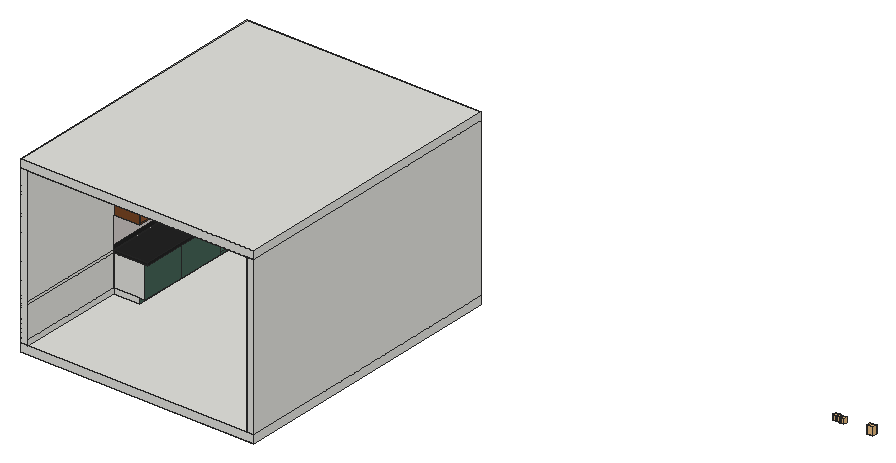
# SketchUp Ruby script. Lengths in inches.
U = 1.inch
M = Sketchup.active_model
def pt(a) = Geom::Point3d.new(a.map { |v| v * U })
def face(e, loops, mat)
  f = e.add_face(loops[0].map { |a| pt(a) })
  loops[1..].each { |l| e.add_face(l.map { |a| pt(a) }).erase! }
  f.material = f.back_material = mat if mat
  f
end
# faces: each face lists its corners as indices into pts; further lists are holes
def faces(e, pts, list, mat = nil) = list.each { |f| face(e, (f[0].is_a?(Array) ? f : [f]).map { |l| l.map { |i| pts[i] } }, mat) }
# xy, xz, yz: faces in a plane at the given z, y or x. An outline is a flat list of corners, or four numbers for a rectangle; further outlines are holes
def ring(l) = l.size == 4 ? [[l[0], l[1]], [l[2], l[1]], [l[2], l[3]], [l[0], l[3]]] : l.each_slice(2).to_a
def flat(e, list, mat, &to3) = list.each { |f| face(e, (f[0].is_a?(Array) ? f : [f]).map { |l| ring(l).map { |u, v| to3.(u, v) } }, mat) }
def xy(e, z, list, mat = nil) = flat(e, list, mat) { |x, y| [x, y, z] }
def xz(e, y, list, mat = nil) = flat(e, list, mat) { |x, z| [x, y, z] }
def yz(e, x, list, mat = nil) = flat(e, list, mat) { |y, z| [x, y, z] }
def lines(e, pts, list) = list.each { |a, b| e.add_line(pt(pts[a]), pt(pts[b])) }
# prism: a flat outline (further loops are holes) pulled along v
def prism(e, loops, v, mat = nil)
  f = face(e, loops, mat); d = Geom::Vector3d.new(v.map { |x| x * U })
  f.pushpull(f.normal.samedirection?(d) ? d.length : -d.length)
end
def box(e, o, s, mat = nil) = prism(e, [[o, [o[0] + s[0], o[1], o[2]], [o[0] + s[0], o[1] + s[1], o[2]], [o[0], o[1] + s[1], o[2]]]], [0, 0, s[2]], mat)
def at(x, y, z, deg = 0) = Geom::Transformation.translation(pt([x, y, z])) * Geom::Transformation.rotation(ORIGIN, Z_AXIS, deg.degrees)
def axes(o, x, y, z) = Geom::Transformation.new([*x, 0, *y, 0, *z, 0, *pt(o).to_a, 1])
def part(name) = M.definitions.add(name)
# library, detail: a bought-in or finely detailed component or shape, given as its bounding box
def library(name, o, s) = part(name).tap { |d| box(d.entities, o, s) }
def detail(e, o, s) = box(e.add_group.entities, o, s)
def put(e, d, t, mat = nil) = e.add_instance(d, t).tap { |i| i.material = mat if mat }
def group(e, t, mat = nil) = e.add_group.tap { |g| g.transformation = t; g.material = mat if mat }.entities
root = M.entities
M.materials.add("4 (5)").color = [147, 109, 57]
M.materials.add("[0012_Bisque]").color = [255, 228, 196]
M.materials.add("[0136_Charcoal]").color = [35, 35, 35]
M.materials.add("[0137_Black]").color = [0, 0, 0]
M.materials.add("[Color C07]").color = [153, 76, 0]
M.materials["[Color C07]"].alpha = 0.27
M.materials.add("[Color G02]").color = [68, 99, 86]
M.materials.add("[Color M08]").color = [30, 30, 30]
M.materials.add("[Tile Hexagon White]").color = [213, 206, 204]
M.materials.add("[Wood Veneer 01]").color = [120, 70, 37]
c1 = part("Group\#46")
prism(c1.entities,[[[0.55,0,1.11],[0.51,0,1.03],[0.44,0,0.97],[0.36,0,0.9375],[0.28,0,0.92],[0.19,0,0.9375],[0.11,0,0.97],[0.05,0,1.03],[0,0,1.11],[0,0,0],[0.55,0,0]]],[0,0.79,0])
c2 = part("Cabinet pull handle")
put(c2.entities,c1,axes([0,1.42,1.36],[0,0,-1],[1,0,0],[0,-1,0]))
g1 = group(c2.entities,at(0,1.42,1.36))
prism(g1,[[[0,-1.28,-0.57],[0,-1.32,-0.53],[0,-1.35,-0.49],[0,-1.38,-0.4375],[0,-1.4,-0.39],[0,-1.41,-0.33],[0,-1.42,-0.28],[0,-1.41,-0.22],[0,-1.4,-0.17],[0,-1.38,-0.11],[0,-1.35,-0.0625],[0,-1.32,-0.02],[0,-1.28,0.02],[0,-1.19,0.02],[0,-1.11,0],[0,-1.03,-0.05],[0,-0.97,-0.11],[0,-0.9375,-0.19],[0,-0.92,-0.28],[0,-0.9375,-0.36],[0,-0.97,-0.44],[0,-1.03,-0.51],[0,-1.11,-0.55],[0,-1.19,-0.57]]],[13.07,0,0])
put(c2.entities,c1,axes([12.28,1.42,1.36],[0,0,-1],[1,0,0],[0,-1,0]))
c3 = library("Food+jars (1)",[-3.15,-4.1,0],[15.4,16.05,11.47])
c4 = library("Stack of bowls \#1",[0,0,0],[8.98,8.99,10.96])
c5 = library("jars",[-134.79,-4.32,0],[83.43,13.28,34.83])
c6 = library("KITCHEN+ITEMS+(3)",[-2.27,-9.02,0],[4.03,10.9,5.45])
c7 = library("filizanka,+spodek+zestaw",[-38.08,-53.17,0],[37.3,56.83,6.3])
c8 = library("Food+jars",[176.18,154.2,55.15],[6.14,23.65,7.76])
c9 = library("Component_12",[0,0,0],[17.72,31.5,20.63])
c10 = library("1045",[78.33,40.52,-0.08],[23.62,20.2,1.2])
c11 = library("PV977NSS_GEProfile",[-17.9375,-27.5625,-0.25],[35.95,27.64,32.08])
c12 = part("Sink basin")
detail(c12.entities,[-0.15,-0.15,0],[19.98,14.07,5.91])
c13 = part("Untitled (26)")
put(c13.entities,c12,at(0.15,0.15,0),"4 (5)")
c14 = library("Group\#21",[-462.66,84.21,613.65],[72.44,72.44,111.8])
c15 = library("Group\#23",[-457.8,68.7,378.69],[103.44,103.46,159.72])
c16 = library("Group\#22",[-210.76,89.58,378.69],[103.46,103.45,159.72])
c17 = library("Group\#24",[-332.7,68.71,378.69],[103.45,103.45,159.72])
c18 = library("Group\#15",[-374.05,84.21,613.65],[72.44,72.44,111.8])
c19 = library("Group\#14",[-289.4,84.22,613.65],[72.44,72.43,111.8])
c20 = library("Group\#13",[-92.73,64.66,378.72],[126.77,111.9,197.69])
c21 = library("Group\#9",[51.24,128.79,378.72],[113.79,95.47,197.69])
c22 = library("Group\#10",[179.9,72.7,378.72],[113.8,95.46,197.69])
c23 = library("Group\#11",[327.72,72.7,378.72],[113.79,95.46,197.69])
c24 = library("Group\#12",[309.63,77.04,613.73],[136.79,86.78,171.39])
c25 = library("Group\#25",[0,0,0],[16.24,2.86,5.88])
xy(root,-6,[[0,0,178.59,216.47]])
xy(root,0,[[0,0,5.86,0,5.86,81.5625,25.86,81.5625,25.86,190.14,5.92,190.07,5.86,210.07,5.86,210.61,172.73,210.61,172.8,190.61,172.73,190.61,172.73,0,178.59,0,178.59,216.47,0,216.47],[5.86,0,172.73,0,172.73,190.61,29.92,190.15,25.86,190.14,25.86,81.5625,5.86,81.5625],[5.92,190.07,25.86,190.14,25.86,210.07,5.86,210.07],[25.86,190.14,25.86,210.07,29.86,210.07,29.92,190.15],[29.92,190.15,172.73,190.61,172.73,210.07,29.86,210.07],
  [172.73,190.61,172.73,210.61,172.8,190.61],[5.86,210.07,29.86,210.15,29.86,210.07],[5.86,210.07,5.86,210.61,29.86,210.61,29.86,210.15],[29.86,210.07,172.73,210.15],[29.86,210.15,172.73,210.15,172.73,210.61],
  [29.86,210.15,29.86,210.61,172.73,210.61]])
xy(root,0.4375,[[29.86,190.15,172.73,190.61,172.73,190.15],[29.86,190.15,172.73,190.61,172.73,210.07,29.86,210.07],[172.73,190.61,172.8,190.61,172.73,210.61,5.86,210.07,172.73,210.07]])
xy(root,4,[[5.86,81.5625,5.86,210.07,5.92,190.07,25.86,190.14,25.86,81.5625],[25.86,81.5625,25.86,190.14,29.86,190.15,29.86,81.5625],[29.86,188.15,172.73,190.15],[5.92,190.07,25.86,190.14,25.86,210.07,5.86,210.07],[25.86,190.14,25.86,210.07,29.86,210.07,29.86,190.15],
  [29.86,190.15,172.73,210.07]])
xy(root,4.67,[[9.42,153.29,29.86,187.48]],"[Color G02]")
xy(root,12.39,[[31.11,188.15,65.58,188.46],[65.58,188.15,101.3,188.46]])
xy(root,12.6875,[[31.11,188.15,65.58,188.46],[65.58,188.15,101.3,188.46]])
xy(root,16,[[9.42,153.29,29.86,187.48]])
xy(root,16.67,[[9.42,153.29,29.86,187.48]],"[Color G02]")
xy(root,20.25,[[31.86,190.15,172.73,210.61]])
xy(root,20.77,[[31.11,188.15,65.58,188.53],[65.58,188.15,101.3,188.46]])
xy(root,21.07,[[31.11,188.15,65.58,188.53],[65.58,188.15,101.3,188.46]])
xy(root,23,[[136.1,188.6,163.66,208.78]])
xy(root,27.33,[[9.42,153.29,29.86,187.48]])
xy(root,28,[[5.86,81.5625,29.86,210.61],[29.86,81.5625,31.86,188.15],[31.86,184.61,172.73,188.15],[29.86,188.15,31.86,190.15],[31.86,188.15,172.73,190.15],
  [29.86,190.15,31.86,210.61]])
xy(root,30,[[[5.86,81.5625,31.86,81.5625,31.86,184.61,172.73,184.61,172.73,210.61,5.86,210.61],[136.1,188.6,163.66,208.78]]],"[0136_Charcoal]")
xy(root,54,[[5.86,81.5625,25.86,210.61],[98.11,197.13,172.73,210.61],[25.86,197.48,60.23,210.61]],"[Wood Veneer 01]")
xy(root,54.4,[[98.11,197.13,98.51,197.14]])
xy(root,54.4,[[98.51,197.13,172.73,197.13,172.73,197.44,172.33,197.44,172.33,212.98,98.51,212.98]],"[Wood Veneer 01]")
xy(root,54.6,[[1.8,82.18,25.86,82.18,25.86,197.14,59.63,197.14,59.63,212.98,1.8,212.98]],"[Wood Veneer 01]")
xy(root,65.38,[[1.8,82.18,25.86,108.82],[1.8,108.82,25.86,136.09],[1.8,136.09,25.86,163.35],[1.8,163.35,25.86,190.61]],"[Wood Veneer 01]")
xy(root,65.4,[[1.8,190.61,59.63,212.98]],"[Wood Veneer 01]")
xy(root,65.6,[[98.51,190.61,117.8,212.98],[117.8,190.61,136.3,212.98],[136.3,190.61,155.11,212.98],[155.11,190.61,172.33,212.98]],"[Wood Veneer 01]")
xy(root,66,[[60.23,190.61,98.11,210.61]])
xy(root,66.67,[[1.8,109.5,25.86,162.67]])
xy(root,66.82,[[98.92,190.61,135.48,212.98]])
xy(root,67.18,[[27.03,190.61,59.06,212.98]])
xy(root,76.6,[[1.8,109.5,25.3,162.67]])
xy(root,77.39,[[98.92,193.17,135.48,212.98]])
xy(root,78,[[1.8,109.5,25.3,162.67],[98.92,193.17,135.48,212.98]])
xy(root,78.8125,[[27.03,192.23,59.06,212.98]])
xy(root,79.375,[[27.03,192.23,59.06,212.98]])
xy(root,88.82,[[27.03,190.61,59.06,212.98]])
xy(root,89.18,[[98.92,190.61,135.48,212.98]])
xy(root,89.33,[[1.8,109.5,25.86,162.67]])
xy(root,90,[[25.86,81.5625,33.3,186.61],[33.3,183.17,33.3,186.61,25.86,186.61,25.86,190.61,172.73,190.61,172.73,183.17]],"[Wood Veneer 01]")
xy(root,92,[[29.86,81.5625,33.3,186.61],[33.3,183.17,172.73,186.61]])
xy(root,120,[[0,0,0,216.47,178.59,216.47,178.59,0,172.73,0,172.73,186.61,29.86,186.61,29.86,81.5625,5.86,81.5625,5.86,0],[5.86,0,5.86,81.5625,29.86,81.5625,29.86,186.61,172.73,186.61,172.73,0]])
xy(root,126,[[0,0,178.59,216.47]])
xz(root,0,[[0,-6,178.59,0],[0,0,5.86,120],[172.73,0,178.59,120],[0,120,178.59,126]])
xz(root,81.5625,[[5.86,0,25.86,4],[5.86,4,29.86,28],[25.86,66,25.86,90,5.86,90,5.86,66.67],[5.86,90,33.3,92],[5.86,92,29.86,120]])
xz(root,81.5625,[[5.86,28,31.86,30]],"[0136_Charcoal]")
xz(root,81.5625,[[5.86,54,25.86,54,25.86,66,5.86,66.67]],"[Wood Veneer 01]")
xz(root,82.18,[[1.8,54.6,25.86,65.38]])
xz(root,109.5,[[1.8,66.67,25.86,76.6],[25.3,76.6,25.86,78],[1.8,78,25.86,89.33]])
xz(root,153.29,[[9.42,4.67,29.86,16],[9.42,16,29.86,16.67],[9.42,16.67,29.86,27.33]])
xz(root,162.67,[[1.8,66.67,25.86,76.6],[25.3,76.6,25.86,78],[1.8,78,25.86,89.33]])
xz(root,183.17,[[33.3,90,172.73,92]],"[Wood Veneer 01]")
xz(root,184.61,[[31.86,28,172.73,30]],"[0137_Black]")
xz(root,186.61,[[33.3,92,33.6,120],[77.48,92,77.78,120],[125.11,92,125.41,120]])
xz(root,186.61,[[29.86,92,33.3,120],[33.6,92,77.48,120],[77.78,92,125.11,120],[125.41,92,172.73,120]],"[0012_Bisque]")
xz(root,187.48,[[9.42,4.67,29.86,16],[9.42,16.67,29.86,27.33]],"[Color G02]")
xz(root,188.15,[[29.86,4,31.11,28],[31.11,4,65.58,12.39],[65.58,4,101.3,12.39],[101.3,4,137.01,28],[137.01,4,172.73,28],
  [31.11,12.6875,65.58,20.77],[65.58,12.6875,101.3,20.77],[31.11,21.07,65.58,28],[65.58,21.07,101.3,28]],"[Color G02]")
xz(root,188.46,[[31.11,12.39,65.58,12.6875],[65.58,12.39,101.3,12.6875],[65.58,20.77,101.3,21.07]])
xz(root,188.53,[[31.11,20.77,65.58,21.07]])
xz(root,188.6,[[136.1,23,163.66,30]])
xz(root,190.15,[[29.86,4,29.86,28,31.86,28,31.86,20.25,172.73,20.25,172.73,4],[31.86,20.25,172.73,28]])
xz(root,190.15,[[29.86,0.4375,172.73,4]],"[Color G02]")
xz(root,190.61,[[1.8,65.38,25.86,65.4],[25.86,65.4,59.63,66],[155.11,66,155.41,90]])
xz(root,190.61,[[60.23,66,98.11,90]],"[0012_Bisque]")
xz(root,190.61,[[136.3,66,155.11,90],[155.41,66,172.73,90]],"[Color G02]")
xz(root,190.61,[[[25.86,66,60.23,90],[27.03,67.18,59.06,88.82]],[[98.11,66,136.3,90],[98.92,66.82,135.48,89.18]]],"[Color M08]")
xz(root,190.61,[[98.51,65.6,172.73,66]],"[Wood Veneer 01]")
xz(root,192.23,[[27.03,78.8125,59.06,79.375]])
xz(root,193.17,[[98.92,77.39,135.48,78]])
xz(root,197.13,[[98.11,54,172.73,54.4]],"[Wood Veneer 01]")
xz(root,197.14,[[98.11,54.4,98.51,54.6]])
xz(root,208.78,[[136.1,23,163.66,30]])
xz(root,210.07,[[5.86,0,25.86,0.4375],[25.86,0,29.86,0.4375],[29.86,0,172.73,0.4375],[5.86,0.4375,25.86,4],[25.86,0.4375,29.86,4],
  [29.86,0.4375,172.73,4]])
xz(root,210.61,[[5.86,0,29.86,28],[29.86,0,172.73,0,172.73,20.25,31.86,20.25,31.86,28,29.86,28],[31.86,20.25,172.73,30],[5.86,28,31.86,30]])
xz(root,210.61,[[5.86,30,172.73,33.57]],"[0136_Charcoal]")
xz(root,210.61,[[5.86,33.57,172.73,33.57,172.73,54,98.11,54,98.11,66,60.23,66,60.23,54,5.86,54]],"[Tile Hexagon White]")
xz(root,212.98,[[98.92,66.82,135.48,77.39],[27.03,67.18,59.06,78.8125],[98.92,78,135.48,89.18],[27.03,79.375,59.06,88.82]])
xz(root,212.98,[[98.51,54.4,172.33,65.6],[1.8,54.6,59.63,65.4]],"[Wood Veneer 01]")
xz(root,216.47,[[0,-6,178.59,0],[0,0,178.59,120],[0,120,178.59,126]])
yz(root,0,[[0,-6,216.47,0],[0,0,216.47,120],[0,120,216.47,126]])
yz(root,1.8,[[109.5,66.67,162.67,76.6],[109.5,78,162.67,89.33]])
yz(root,1.8,[[82.18,54.6,212.98,54.6,212.98,65.4,190.61,65.4,190.61,65.38,82.18,65.38]],"[Wood Veneer 01]")
yz(root,5.86,[[0,0,81.5625,4],[210.07,0,210.07,4,81.5625,4,81.5625,28,210.61,28,210.61,0],[0,4,81.5625,28],[0,28,81.5625,30],[81.5625,28,210.61,30],
  [0,30,81.5625,120]])
yz(root,5.86,[[81.5625,30,210.61,33.57]],"[0136_Charcoal]")
yz(root,5.86,[[81.5625,33.57,210.61,54]],"[Tile Hexagon White]")
yz(root,9.42,[[153.29,4.67,187.48,16],[153.29,16.67,187.48,27.33]])
yz(root,25.3,[[109.5,76.6,162.67,78]])
yz(root,25.86,[[81.5625,66,108.82,90],[163.35,66,190.61,90]],"[0012_Bisque]")
yz(root,25.86,[[81.5625,0,210.07,4]],"[Color G02]")
yz(root,25.86,[[[108.82,66,163.35,90],[109.5,66.67,162.67,89.33]]],"[Color M08]")
yz(root,25.86,[[81.5625,54,190.61,54,190.61,54.6,82.18,54.6,82.18,65.38,190.61,65.38,190.61,66,81.5625,66],[190.61,54,197.48,54,197.14,54.6,190.61,54.6]],"[Wood Veneer 01]")
yz(root,27.03,[[190.61,67.18,212.98,67.18,212.98,78.8125,192.23,78.8125,192.23,79.375,212.98,79.375,212.98,88.82,190.61,88.82]])
yz(root,29.86,[[210.07,0,210.07,4,190.15,4,190.15,28,210.61,28,210.61,0],[190.15,0.4375,210.07,4],[188.15,4,190.15,28],[116.58,92,116.88,120],[151.59,92,151.89,120]])
yz(root,29.86,[[81.5625,92,116.58,120],[116.88,92,151.59,120],[151.89,92,186.61,120]],"[0012_Bisque]")
yz(root,29.86,[[81.5625,4,117.09,28],[117.09,4,152.62,28],[[152.62,4,188.15,28],[153.29,4.67,187.48,16],[153.29,16.67,187.48,27.33]]],"[Color G02]")
yz(root,31.11,[[188.15,12.39,188.46,12.6875],[188.15,20.77,188.53,21.07]])
yz(root,31.86,[[190.15,20.25,210.61,28]])
yz(root,31.86,[[81.5625,28,184.61,30]],"[0136_Charcoal]")
yz(root,33.3,[[81.5625,90,183.17,92]],"[Wood Veneer 01]")
yz(root,59.06,[[190.61,67.18,190.61,88.82,212.98,88.82,212.98,79.375,192.23,79.375,192.23,78.8125,212.98,78.8125,212.98,67.18]])
yz(root,59.63,[[197.14,54.6,190.95,65.4,212.98,65.4,212.98,54.6],[190.61,65.4,190.95,65.4,190.61,66]])
yz(root,60.23,[[197.48,54,210.61,54,210.61,66,190.61,66,197.14,54.6]],"[Wood Veneer 01]")
yz(root,65.58,[[188.46,20.77,188.53,21.07]])
yz(root,98.11,[[197.13,54,197.13,54.4,197.14,54.4,197.14,54.6,190.61,66,210.61,66,210.61,54]],"[Wood Veneer 01]")
yz(root,98.51,[[190.61,65.6,190.61,66,190.84,65.6]])
yz(root,98.51,[[197.14,54.4,212.98,54.4,212.98,65.6,190.84,65.6,197.14,54.6]],"[Wood Veneer 01]")
yz(root,98.92,[[190.61,66.82,212.98,77.39],[190.61,77.39,193.17,78],[193.17,77.39,212.98,78],[190.61,78,212.98,89.18]])
yz(root,101.3,[[188.15,12.39,188.46,12.6875],[188.15,20.77,188.46,21.07]])
yz(root,135.48,[[190.61,66.82,212.98,77.39],[190.61,77.39,193.17,78],[190.61,78,212.98,89.18]])
yz(root,136.1,[[188.6,23,208.78,30]])
yz(root,163.66,[[188.6,23,208.78,30]])
yz(root,172.33,[[197.44,54.4,190.61,65.6,212.98,65.6,212.98,54.4]],"[Wood Veneer 01]")
yz(root,172.73,[[0,0,0,120,186.61,120,186.61,92,183.17,92,183.17,90,190.61,90,190.61,65.6,197.44,54.4,197.13,54.4,197.13,54,210.61,54,210.61,30,184.61,30,184.61,28,188.15,28,188.15,4,190.15,4,190.15,0.4375,210.07,0.4375,210.07,0],[210.07,0,210.61,0,210.61,20.25,190.15,20.25,190.15,4,210.07,4],[190.15,0.4375,210.07,4],[188.15,4,190.15,28],[190.15,20.25,190.15,28,184.61,28,184.61,30,210.61,30,210.61,20.25]])
yz(root,178.59,[[0,-6,216.47,0],[0,0,216.47,120],[0,120,216.47,126]])
p = [[5.86,210.07,4],[5.86,210.07,0.4375],[5.86,210.07,0],[5.92,190.07,0],[5.92,190.07,4],[172.73,190.61,0],
  [172.8,190.61,0],[172.8,190.61,0.4375],[172.73,190.61,0.4375],[29.86,190.15,0.4375],[29.86,190.15,4],[25.86,190.14,4],
  [25.86,190.14,0],[29.92,190.15,0],[172.73,210.61,0],[172.73,210.61,0.4375],[29.86,210.15,0],[60.23,197.48,54],
  [60.23,197.14,54.6],[59.63,197.14,54.6],[25.86,197.14,54.6],[25.86,197.48,54],[172.33,190.61,65.6],[172.33,197.44,54.4],
  [172.73,197.44,54.4],[172.73,190.61,65.6],[60.23,190.61,66],[59.63,190.61,66],[59.63,190.95,65.4],[98.11,190.61,66],
  [98.11,197.14,54.6],[98.51,197.14,54.6],[98.51,190.84,65.6],[98.51,190.61,66]]
faces(root,p,[[0,1,2,3,4],[14,15,7,6],[14,16,2,1,15]])
faces(root,p,[[5,6,7,8,9,10,11,4,3,12,13]],"[Color G02]")
faces(root,p,[[17,18,19,20,21],[22,23,24,25],[18,26,27,28,19],[29,30,31,32,33]],"[Wood Veneer 01]")
put(root,c2,axes([45.91,187.32,19.48],[0.5865,0,0],[0,0.5865,0],[0,0,0.5865]))
put(root,c2,axes([45.17,186.73,10.22],[0.63,0,0],[0,1,0],[0,0,1]))
put(root,c2,axes([79.47,187.32,19.48],[0.5865,0,0],[0,0.5865,0],[0,0,0.5865]))
put(root,c2,axes([78.74,186.73,10.22],[0.63,0,0],[0,1,0],[0,0,1]))
put(root,c2,axes([47.87,185.19,92.49],[0.63,0,0],[0,1,0],[0,0,1]))
put(root,c2,axes([97.56,185.19,92.49],[0.63,0,0],[0,1,0],[0,0,1]))
put(root,c2,axes([145.68,185.19,92.49],[0.63,0,0],[0,1,0],[0,0,1]))
put(root,c2,axes([31.28,95.85,92.27],[0,0.63,0],[-1,0,0],[0,0,1]))
put(root,c2,axes([31.28,128.35,92.27],[0,0.63,0],[-1,0,0],[0,0,1]))
put(root,c2,axes([31.28,162.6,92.27],[0,0.63,0],[-1,0,0],[0,0,1]))
put(root,c3,axes([122.77,197.4,66.82],[0.83,0,0],[0,0.83,0],[0,0,0.83]))
put(root,c4,at(104.48,193.17,78))
put(root,c5,axes([143.84,198.51,54.4],[0.32,0,0],[0,0.32,0],[0,0,0.32]))
put(root,c6,axes([154.57,203.04,54.4],[0,-3.37,0],[2.1,0,0],[0,0,1]))
put(root,c7,axes([56.9,190.15,67.18],[0,-0.59,0],[0.59,0,0],[0,0,0.59]),"[Color C07]")
put(root,c4,at(44.19,192.23,78.8125))
put(root,c8,at(-154.375,-44.81,24.76))
put(root,c9,axes([133.2,210.61,20.81],[0,-1.33764,0],[0.9672,0,0],[0,0,1]))
put(root,c10,axes([-12.38,147.67,30.16],[1,0,0],[0,1,0],[0,0,2]))
put(root,c11,at(79.8,210.61,61.38))
put(root,c13,at(29.86,162.72,4.67,90))
put(root,c13,at(29.86,160.71,16.67,90))
g2 = group(root,at(25.86,190.61,66))
xy(g2,0,[[0,0,33.77,1.625],[33.77,0,34.375,1.625]])
xy(g2,1.18,[[1.18,0,33.2,0.8125],[1.18,0.8125,33.2,1.625]])
xy(g2,22.82,[[1.18,0,33.2,0.8125],[1.18,0.8125,33.2,1.625]])
xy(g2,24,[[0,0,34.375,1.625]])
xz(g2,0,[[[0,0,34.375,24],[1.18,1.18,33.2,22.82]]])
xz(g2,0.8125,[[1.18,1.18,33.2,22.82]],"[Color C07]")
xz(g2,1.625,[[[0,0,34.375,24],[1.18,1.18,33.2,22.82]]])
yz(g2,0,[[0,0,1.625,24]])
yz(g2,1.18,[[0,1.18,0.8125,22.82],[0.8125,1.18,1.625,22.82]])
yz(g2,33.2,[[0,1.18,0.8125,22.82],[0.8125,1.18,1.625,22.82]])
yz(g2,34.375,[[0,0,1.625,24]])
put(root,c14,axes([459.78,217.69,-14.16],[0.0341,0,0],[0,0.0341,0],[0,0,0.0341]))
put(root,c15,axes([25.66,169.27,36.84],[0,0.04672,0],[-0.04672,0,0],[0,0,0.04672]))
put(root,c16,axes([25.66,169.27,36.84],[0,0.04672,0],[-0.04672,0,0],[0,0,0.04672]))
put(root,c17,axes([25.66,169.27,36.84],[0,0.04672,0],[-0.04672,0,0],[0,0,0.04672]))
put(root,c18,axes([459.78,217.69,-14.16],[0.0341,0,0],[0,0.0341,0],[0,0,0.0341]))
put(root,c19,axes([459.78,217.69,-14.16],[0.0341,0,0],[0,0.0341,0],[0,0,0.0341]))
put(root,c20,axes([25.4375,120.65,53.76],[0,0.0341,0],[-0.0341,0,0],[0,0,0.0341]))
put(root,c21,axes([28.0625,120.65,53.76],[0,0.0341,0],[-0.0341,0,0],[0,0,0.0341]))
put(root,c22,axes([25.4375,120.65,53.76],[0,0.0341,0],[-0.0341,0,0],[0,0,0.0341]))
put(root,c23,axes([25.4375,120.65,53.76],[0,0.0341,0],[-0.0341,0,0],[0,0,0.0341]))
put(root,c24,axes([459.78,217.69,-14.16],[0.0341,0,0],[0,0.0341,0],[0,0,0.0341]))
put(root,c14,axes([56.52,196.95,12.74],[0.07229,0,0],[0,0.0341,0],[0,0,0.0682]))
put(root,c19,axes([56.52,196.95,12.74],[0.07229,0,0],[0,0.0341,0],[0,0,0.0682]))
put(root,c18,axes([56.52,196.95,12.74],[0.07229,0,0],[0,0.0341,0],[0,0,0.0682]))
put(root,c25,axes([22.92,167.2,54.6],[0,1.5,0],[-1.5,0,0],[0,0,1.5]))
put(root,c14,axes([74.77,196.95,12.74],[0.07229,0,0],[0,0.0341,0],[0,0,0.0682]))
put(root,c19,axes([74.77,196.95,12.74],[0.07229,0,0],[0,0.0341,0],[0,0,0.0682]))
put(root,c18,axes([74.77,196.95,12.74],[0.07229,0,0],[0,0.0341,0],[0,0,0.0682]))
put(root,c18,axes([25.51,150.48,12.75],[0.00429,0.07216,0],[-0.03404,0.00202,0],[0,0,0.0682]))
put(root,c19,axes([25.51,150.48,12.75],[0.00429,0.07216,0],[-0.03404,0.00202,0],[0,0,0.0682]))
put(root,c14,axes([25.51,150.48,12.75],[0.00429,0.07216,0],[-0.03404,0.00202,0],[0,0,0.0682]))
put(root,c14,axes([24.42,132.27,12.75],[0.00429,0.07216,0],[-0.03404,0.00202,0],[0,0,0.0682]))
put(root,c19,axes([24.42,132.27,12.75],[0.00429,0.07216,0],[-0.03404,0.00202,0],[0,0,0.0682]))
put(root,c18,axes([24.42,132.27,12.75],[0.00429,0.07216,0],[-0.03404,0.00202,0],[0,0,0.0682]))
g3 = group(root,at(24.17,108.82,66))
xy(g3,0,[[0,0,1.6875,54.52]])
xy(g3,0.67,[[0,0.67,0.84,53.85],[0.84,0.67,1.6875,53.85]])
xy(g3,23.33,[[0,0.67,0.84,53.85],[0.84,0.67,1.6875,53.85]])
xy(g3,24,[[0,0,1.6875,54.52]])
xz(g3,0,[[0,0,1.6875,24]])
xz(g3,0.67,[[0,0.67,0.84,10.6],[0.84,0.67,1.6875,10.6],[0,10.6,0.84,12],[0.84,10.6,1.6875,12],[0,12,0.84,23.33],
  [0.84,12,1.6875,23.33]])
xz(g3,53.85,[[0,0.67,0.84,10.6],[0.84,0.67,1.6875,10.6],[0,10.6,0.84,12],[0.84,10.6,1.6875,12],[0,12,0.84,23.33],
  [0.84,12,1.6875,23.33]])
xz(g3,54.52,[[0,0,1.6875,24]])
yz(g3,0,[[[0,0,54.52,24],[0.67,0.67,53.85,23.33]]])
yz(g3,0.84,[[0.67,0.67,53.85,23.33]],"[Color C07]")
yz(g3,1.6875,[[[0,0,54.52,24],[0.67,0.67,53.85,23.33]]])
g4 = group(root,at(98.11,190.61,66))
xy(g4,0,[[0,0,0.4,1.125],[0.4,0,38.1875,1.125]])
xy(g4,0.82,[[0.82,0,37.37,0.5625],[0.82,0.5625,37.37,1.125]])
xy(g4,23.18,[[0.82,0,37.37,0.5625],[0.82,0.5625,37.37,1.125]])
xy(g4,24,[[0,0,38.1875,1.125]])
xz(g4,0,[[[0,0,38.1875,24],[0.82,0.82,37.37,23.18]]])
xz(g4,0.5625,[[0.82,0.82,37.37,23.18]],"[Color C07]")
xz(g4,1.125,[[[0,0,38.1875,24],[0.82,0.82,37.37,23.18]]])
yz(g4,0,[[0,0,1.125,24]])
yz(g4,0.82,[[0,0.82,0.5625,11.39],[0.5625,0.82,1.125,11.39],[0,11.39,0.5625,12],[0.5625,11.39,1.125,12],[0,12,0.5625,23.18],
  [0.5625,12,1.125,23.18]])
yz(g4,37.37,[[0,0.82,0.5625,11.39],[0.5625,0.82,1.125,11.39],[0,11.39,0.5625,12],[0.5625,11.39,1.125,12],[0,12,0.5625,23.18],
  [0.5625,12,1.125,23.18]])
yz(g4,38.1875,[[0,0,1.125,24]])
